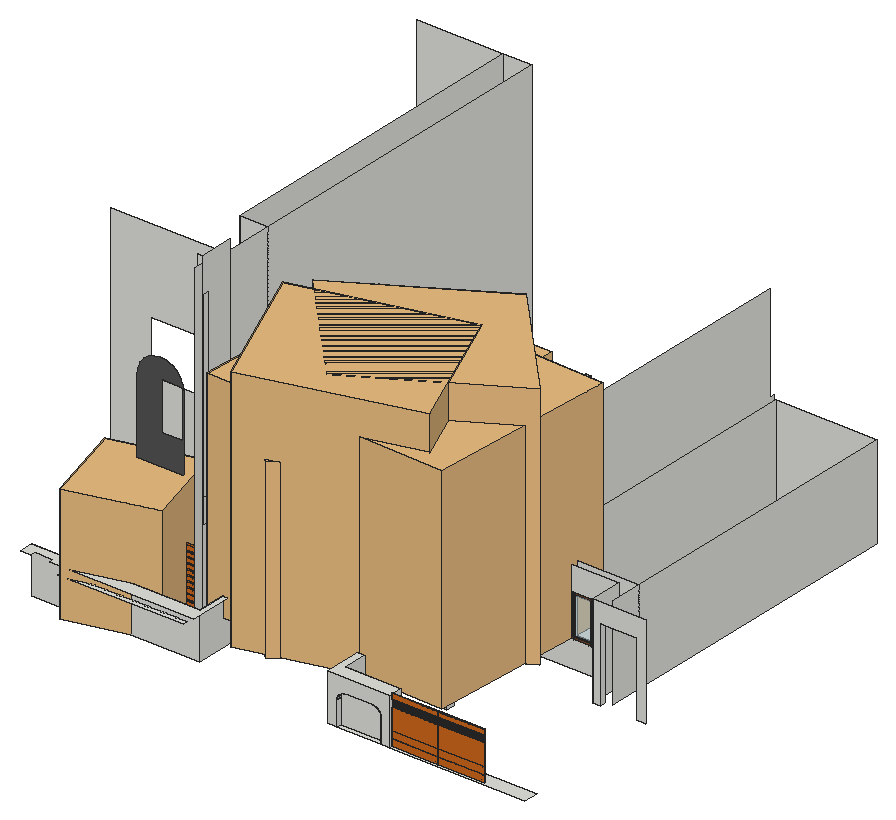
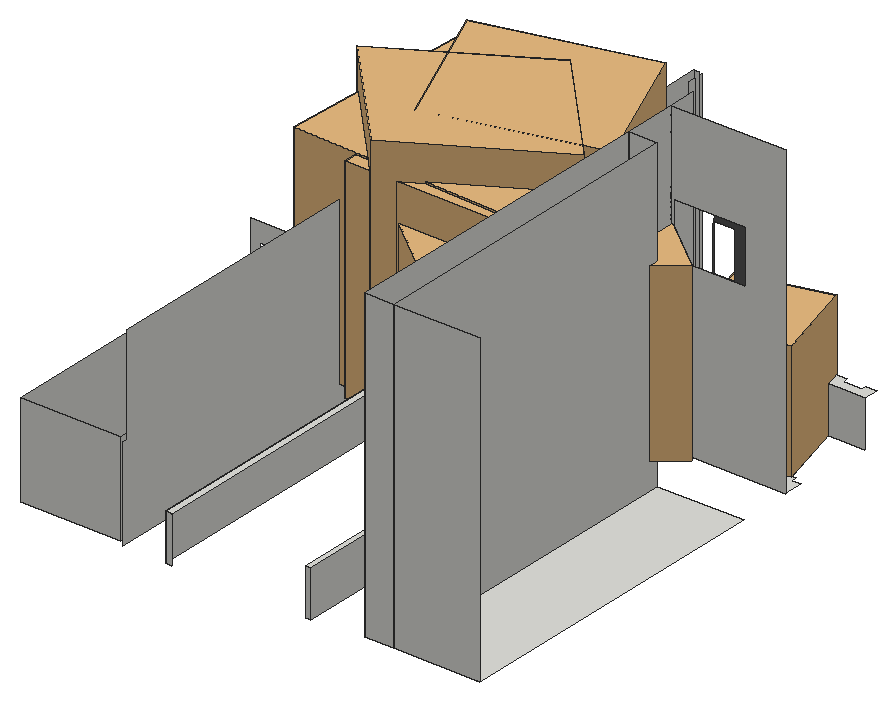
# SketchUp Ruby script. Lengths in inches.
U = 1.inch
M = Sketchup.active_model
def pt(a) = Geom::Point3d.new(a.map { |v| v * U })
def face(e, loops, mat)
  f = e.add_face(loops[0].map { |a| pt(a) })
  loops[1..].each { |l| e.add_face(l.map { |a| pt(a) }).erase! }
  f.material = f.back_material = mat if mat
  f
end
# faces: each face lists its corners as indices into pts; further lists are holes
def faces(e, pts, list, mat = nil) = list.each { |f| face(e, (f[0].is_a?(Array) ? f : [f]).map { |l| l.map { |i| pts[i] } }, mat) }
# xy, xz, yz: faces in a plane at the given z, y or x. An outline is a flat list of corners, or four numbers for a rectangle; further outlines are holes
def ring(l) = l.size == 4 ? [[l[0], l[1]], [l[2], l[1]], [l[2], l[3]], [l[0], l[3]]] : l.each_slice(2).to_a
def flat(e, list, mat, &to3) = list.each { |f| face(e, (f[0].is_a?(Array) ? f : [f]).map { |l| ring(l).map { |u, v| to3.(u, v) } }, mat) }
def xy(e, z, list, mat = nil) = flat(e, list, mat) { |x, y| [x, y, z] }
def xz(e, y, list, mat = nil) = flat(e, list, mat) { |x, z| [x, y, z] }
def yz(e, x, list, mat = nil) = flat(e, list, mat) { |y, z| [x, y, z] }
def lines(e, pts, list) = list.each { |a, b| e.add_line(pt(pts[a]), pt(pts[b])) }
# prism: a flat outline (further loops are holes) pulled along v
def prism(e, loops, v, mat = nil)
  f = face(e, loops, mat); d = Geom::Vector3d.new(v.map { |x| x * U })
  f.pushpull(f.normal.samedirection?(d) ? d.length : -d.length)
end
def box(e, o, s, mat = nil) = prism(e, [[o, [o[0] + s[0], o[1], o[2]], [o[0] + s[0], o[1] + s[1], o[2]], [o[0], o[1] + s[1], o[2]]]], [0, 0, s[2]], mat)
def at(x, y, z, deg = 0) = Geom::Transformation.translation(pt([x, y, z])) * Geom::Transformation.rotation(ORIGIN, Z_AXIS, deg.degrees)
def axes(o, x, y, z) = Geom::Transformation.new([*x, 0, *y, 0, *z, 0, *pt(o).to_a, 1])
def part(name) = M.definitions.add(name)
# library, detail: a bought-in or finely detailed component or shape, given as its bounding box
def library(name, o, s) = part(name).tap { |d| box(d.entities, o, s) }
def detail(e, o, s) = box(e.add_group.entities, o, s)
def put(e, d, t, mat = nil) = e.add_instance(d, t).tap { |i| i.material = mat if mat }
def group(e, t, mat = nil) = e.add_group.tap { |g| g.transformation = t; g.material = mat if mat }.entities
root = M.entities
M.materials.add("[0041_Chocolate]").color = [210, 105, 30]
M.materials.add("[Color M06]").color = [84, 84, 84]
M.materials.add("[Translucent Glass Safety]").color = [204, 235, 244]
M.materials["[Translucent Glass Safety]"].alpha = 0.5
M.materials.add("[Wood Veneer 01]").color = [120, 70, 37]
M.materials.add("[Wood Veneer 01]2").color = [94, 55, 29]
c1 = library("Palm tree",[-4.09,-4.52,0],[193.52,193.51,258.93])
c2 = part("Palm+Tree")
put(c2.entities,c1,at(25.51,-21.81,0,15))
c3 = library("Group\#287",[-33.32,-34.9375,32.67],[162.87,159.66,128.34])
c4 = library("Group\#288",[-10.45,-6.67,0],[121.7,116.61,164.95])
c5 = library("Group\#286",[-10.45,-6.67,0],[121.7,116.61,164.95])
c6 = library("Group\#284",[-10.45,-6.67,0],[121.7,116.61,164.95])
c7 = library("Group\#283",[-33.32,-34.9375,32.67],[162.87,159.66,128.34])
c8 = library("Group\#285",[-33.32,-34.9375,81.35],[162.87,159.66,79.66])
c9 = library("Group\#282",[-33.32,-34.9375,77.91],[162.87,159.66,83.1])
c10 = part("Palem Elek")
put(c10.entities,c3,axes([92.2,20.3,-29.73],[0.70711,0.70711,0],[-0.70711,0.70711,0],[0,0,0.91208]))
put(c10.entities,c4,axes([60.27,20.78,0],[1,0,0],[0,1,0],[0,0,0.85762]))
put(c10.entities,c5,at(25.45,60.83,0,-53.5))
put(c10.entities,c6,at(84.4375,135.48,0,-161.4))
put(c10.entities,c7,axes([38.54,105.7,-36.19],[-0.04013,-0.99919,0],[0.99919,-0.04013,0],[0,0,1.11001]))
put(c10.entities,c8,axes([57.15,96.51,-54.45],[-0.02003,-0.49872,0.02965],[0.4996,-0.02007,0],[0.00123,0.03065,0.51628]))
put(c10.entities,c9,axes([74.94,50.39,-54.06],[0.40095,0.29715,0.03075],[-0.29654,0.38966,0.10114],[0.04012,-0.11026,0.54246]))
c11 = part("palem elek\#1")
put(c11.entities,c10,at(-81.14,-74.56,-0.83))
c12 = part("Coqueiro")
put(c12.entities,c11,axes([83.17,89.39,9.5625],[0,1.1016,0],[-1.377,0,0],[0,0,1.39284]))
c13 = part("Slatted screen panel")
xy(c13.entities,0,[[0,0,255.91,1.97]],"[Wood Veneer 01]2")
xy(c13.entities,16.54,[[0,1.18,255.91,1.97]],"[Wood Veneer 01]2")
xy(c13.entities,16.93,[[0,0,255.91,1.18]],"[Wood Veneer 01]2")
xy(c13.entities,17.78,[[0,0,255.91,1.18]],"[Wood Veneer 01]2")
xy(c13.entities,34.45,[[0,0,255.91,1.18]],"[Wood Veneer 01]2")
xy(c13.entities,35.07,[[0,0,255.91,1.18]],"[Wood Veneer 01]2")
xy(c13.entities,89.37,[[0,0,255.91,1.97]],"[Wood Veneer 01]2")
xy(c13.entities,92.91,[[0,0,255.91,1.97]],"[Wood Veneer 01]2")
xy(c13.entities,94.49,[[0,0,255.91,1.97]],"[Wood Veneer 01]2")
xy(c13.entities,97.64,[[0,0,255.91,1.97]],"[Wood Veneer 01]2")
xy(c13.entities,99.21,[[0,0,255.91,1.97]],"[Wood Veneer 01]2")
xy(c13.entities,102.36,[[0,0,255.91,1.97]],"[Wood Veneer 01]2")
xy(c13.entities,103.9375,[[0,0,255.91,1.97]],"[Wood Veneer 01]2")
xy(c13.entities,107.48,[[0,0,255.91,1.97]],"[Wood Veneer 01]2")
xy(c13.entities,119.29,[[0,0,255.91,1.97]],"[Wood Veneer 01]2")
xz(c13.entities,0,[[0,0,255.91,16.93],[0,17.78,255.91,34.45],[0,35.07,255.91,89.37],[0,92.91,255.91,94.49],[0,97.64,255.91,99.21],
  [0,102.36,255.91,103.9375],[0,107.48,255.91,119.29]],"[0041_Chocolate]")
xz(c13.entities,1.18,[[0,16.54,255.91,16.93],[0,16.93,255.91,17.78],[0,34.45,255.91,35.07]],"[Wood Veneer 01]2")
xz(c13.entities,1.97,[[0,0,255.91,1.57],[0,1.57,255.91,5.51],[0,5.51,255.91,7.09],[0,7.09,255.91,11.8125],[0,11.8125,255.91,16.54],
  [0,16.54,255.91,19.69],[0,19.69,255.91,89.37],[0,92.91,255.91,94.49],[0,97.64,255.91,99.21],[0,102.36,255.91,103.9375],
  [0,107.48,255.91,109.84],[0,109.84,255.91,119.29]],"[Wood Veneer 01]2")
yz(c13.entities,0,[[0,0,1.97,1.57],[0,1.57,1.97,5.51],[0,5.51,1.97,7.09],[0,7.09,1.97,11.8125],[0,11.8125,0,16.93,1.18,16.93,1.18,16.54,1.97,16.54,1.97,11.8125],
  [1.18,16.54,1.97,19.69],[0,17.78,0,34.45,1.18,34.45,1.18,35.07,0,35.07,0,89.37,1.97,89.37,1.97,19.69,1.18,19.69,1.18,17.78],[0,92.91,1.97,94.49],[0,97.64,1.97,99.21],[0,102.36,1.97,103.9375],
  [0,107.48,1.97,109.84],[0,109.84,1.97,119.29]],"[Wood Veneer 01]2")
yz(c13.entities,255.91,[[0,0,1.97,1.57],[0,1.57,1.97,5.51],[0,5.51,1.97,7.09],[0,7.09,1.97,11.8125],[0,11.8125,1.97,11.8125,1.97,16.54,1.18,16.54,1.18,16.93,0,16.93],
  [1.18,16.54,1.97,19.69],[0,17.78,1.18,17.78,1.18,19.69,1.97,19.69,1.97,89.37,0,89.37,0,35.07,1.18,35.07,1.18,34.45,0,34.45],[0,92.91,1.97,94.49],[0,97.64,1.97,99.21],[0,102.36,1.97,103.9375],
  [0,107.48,1.97,109.84],[0,109.84,1.97,119.29]],"[Wood Veneer 01]2")
p = [[255.91,1.97,103.9375],[255.91,1.97,107.48],[0,1.97,107.48],[0,1.97,103.9375],[0,1.97,92.91],[0,1.97,89.37],
  [255.91,1.97,99.21],[255.91,1.97,102.36],[255.91,1.97,89.37],[255.91,1.97,92.91],[0,1.97,97.64],[0,1.97,94.49],
  [0,1.97,102.36],[0,1.97,99.21],[255.91,1.97,94.49],[255.91,1.97,97.64],[240.94,0,5.51],[240.94,1.97,5.51]]
lines(c13.entities,p,[[0,1],[2,3],[4,5],[6,7],[8,9],[10,11],[12,13],[14,15],[16,17]])
c14 = part("Group\#3")
g1 = group(c14.entities,at(0,0,0))
xy(g1,0,[[0,0,6,48]],"[Wood Veneer 01]")
xy(g1,4,[[0,4,1.8125,44],[1.8125,4,6,44]])
xy(g1,80,[[0,4,1.8125,44],[1.8125,4,6,44]])
xy(g1,84,[[0,0,6,48]],"[Wood Veneer 01]")
xz(g1,0,[[0,0,6,84]],"[Wood Veneer 01]")
xz(g1,4,[[0,4,1.8125,80],[1.8125,4,6,80]])
xz(g1,44,[[0,4,1.8125,80],[1.8125,4,6,80]])
xz(g1,48,[[0,0,6,84]],"[Wood Veneer 01]")
yz(g1,0,[[[0,0,48,84],[4,4,44,80]]],"[Wood Veneer 01]")
yz(g1,1.8125,[[4,4,44,80]],"[Translucent Glass Safety]")
yz(g1,6,[[[0,0,48,84],[4,4,44,80]]],"[Wood Veneer 01]")
g2 = group(c14.entities,at(0,48,0))
xy(g2,0,[[0,0,6,48]],"[Wood Veneer 01]")
xy(g2,4,[[0,4,1.8125,44],[1.8125,4,6,44]])
xy(g2,80,[[0,4,1.8125,44],[1.8125,4,6,44]])
xy(g2,84,[[0,0,6,48]],"[Wood Veneer 01]")
xz(g2,0,[[0,0,6,84]],"[Wood Veneer 01]")
xz(g2,4,[[0,4,1.8125,80],[1.8125,4,6,80]])
xz(g2,44,[[0,4,1.8125,80],[1.8125,4,6,80]])
xz(g2,48,[[0,0,6,84]],"[Wood Veneer 01]")
yz(g2,0,[[[0,0,48,84],[4,4,44,80]]],"[Wood Veneer 01]")
yz(g2,1.8125,[[4,4,44,80]],"[Translucent Glass Safety]")
yz(g2,6,[[[0,0,48,84],[4,4,44,80]]],"[Wood Veneer 01]")
xy(root,6.125,[[1898.05,198.625,1954.92,204.875],[1965.86,198.625,2140.66,217.125],[1547.71,280.47,1643.23,280.47,1643.23,292.45,1642.35,292.45,1642.35,302.0625,1547.71,302.0625],[1643.23,280.47,1649.14,292.45],[1547.21,292.45,1547.71,302.46],
  [1642.35,292.45,1643.23,302.46],[1643.23,292.45,1650.02,302.46],[1949.9,294.33,1962.9,305.58],[1547.71,302.0625,1642.35,302.46],[1547.71,302.46,1547.71,305.58,1507.74,305.58,1507.74,312.8125,1496.21,312.8125,1496.21,336.27,1643.23,336.27,1643.23,302.46],
  [1547.71,302.46,1547.71,305.58,1507.74,305.58,1507.74,312.8125,1547.71,312.8125,1547.71,305.58,1643.23,305.58,1643.23,302.46],[1547.21,302.46,1547.71,305.58],[1643.23,302.46,1650.02,305.58],[1643.23,305.58,1650.02,336.27],[1496.21,336.27,1643.23,337.5625],
  [1495.03,406.38,1606.23,830.91],[1606.23,406.38,1643.23,830.91],[1957.13,448.51,2087.21,830.91]])
xy(root,11.08,[[1547.71,280.47,1649.14,281.47]],"[0041_Chocolate]")
xy(root,13.1875,[[1547.71,280.47,1649.14,281.47]],"[0041_Chocolate]")
xy(root,18.14,[[1547.71,280.47,1649.14,281.47]],"[0041_Chocolate]")
xy(root,20.25,[[1547.71,280.47,1649.14,281.47]],"[0041_Chocolate]")
xy(root,25.2,[[1547.71,280.47,1649.14,281.47]],"[0041_Chocolate]")
xy(root,27.3125,[[1547.71,280.47,1649.14,281.47]],"[0041_Chocolate]")
xy(root,32.27,[[1547.71,280.47,1649.14,281.47]],"[0041_Chocolate]")
xy(root,34.375,[[1547.71,280.47,1649.14,281.47]],"[0041_Chocolate]")
xy(root,39.33,[[1547.71,280.47,1649.14,281.47]],"[0041_Chocolate]")
xy(root,40.13,[[1985.87,439.98,2033.5,448.51]])
xy(root,41.4375,[[1547.71,280.47,1649.14,281.47]],"[0041_Chocolate]")
xy(root,46.39,[[1547.71,280.47,1649.14,281.47]],"[0041_Chocolate]")
xy(root,48,[[1908.98,198.625,1943.43,204.875]])
xy(root,48.5,[[1547.71,280.47,1649.14,281.47]],"[0041_Chocolate]")
xy(root,53.45,[[1547.71,280.47,1649.14,281.47]],"[0041_Chocolate]")
xy(root,55.1875,[[1539,198.625,1539,203.875,1540.625,203.875,1540.625,204.875,1541.375,204.875,1541.375,203.875,1544.625,203.875,1544.625,204.875,1545.375,204.875,1545.375,203.875,1548.625,203.875,1548.625,204.875,1549.375,204.875,1549.375,203.875,1552.625,203.875,1552.625,204.875,1553.375,204.875,1553.375,203.875,1556.625,203.875,1556.625,204.875,1557.375,204.875,1557.375,203.875,1560.625,203.875,1560.625,204.875,1561.375,204.875,1561.375,203.875,1564.625,203.875,1564.625,204.875,1565.375,204.875,1565.375,203.875,1568.625,203.875,1568.625,204.875,1569.375,204.875,1569.375,203.875,1572.625,203.875,1572.625,204.875,1573.375,204.875,1573.375,203.875,1576.625,203.875,1576.625,204.875,1577.375,204.875,1577.375,203.875,1580.625,203.875,1580.625,204.875,1581.375,204.875,1581.375,203.875,1584.625,203.875,1584.625,204.875,1585.375,204.875,1585.375,203.875,1588.625,203.875,1588.625,204.875,1589.375,204.875,1589.375,203.875,1592.625,203.875,1592.625,204.875,1593.375,204.875,1593.375,203.875,1596.625,203.875,1596.625,204.875,1597.375,204.875,1597.375,203.875,1600.625,203.875,1600.625,204.875,1601.375,204.875,1601.375,203.875,1604.625,203.875,1604.625,204.875,1605.375,204.875,1605.375,203.875,1608.625,203.875,1608.625,204.875,1609.375,204.875,1609.375,203.875,1612.625,203.875,1612.625,204.875,1613.375,204.875,1613.375,203.875,1616.625,203.875,1616.625,204.875,1617.375,204.875,1617.375,203.875,1620.625,203.875,1620.625,204.875,1621.375,204.875,1621.375,203.875,1624.625,203.875,1624.625,204.875,1625.375,204.875,1625.375,203.875,1628.625,203.875,1628.625,204.875,1629.375,204.875,1629.375,203.875,1632.625,203.875,1632.625,204.875,1633.375,204.875,1633.375,203.875,1636.625,203.875,1636.625,204.875,1637.375,204.875,1637.375,203.875,1640.625,203.875,1640.625,204.875,1641.375,204.875,1641.375,203.875,1644.625,203.875,1644.625,204.875,1645.375,204.875,1645.375,203.875,1648.625,203.875,1648.625,204.875,1649.375,204.875,1649.375,203.875,1652.625,203.875,1652.625,204.875,1653.375,204.875,1653.375,203.875,1656.625,203.875,1656.625,204.875,1657.375,204.875,1657.375,203.875,1660.625,203.875,1660.625,204.875,1661.375,204.875,1661.375,203.875,1664.625,203.875,1664.625,204.875,1665.375,204.875,1665.375,203.875,1668.625,203.875,1668.625,204.875,1669.375,204.875,1669.375,203.875,1672.625,203.875,1672.625,204.875,1673.375,204.875,1673.375,203.875,1676.625,203.875,1676.625,204.875,1677.375,204.875,1677.375,203.875,1680.625,203.875,1680.625,204.875,1681.375,204.875,1681.375,203.875,1684.625,203.875,1684.625,204.875,1685.375,204.875,1685.375,203.875,1688.625,203.875,1688.625,204.875,1689.375,204.875,1689.375,203.875,1692.625,203.875,1692.625,204.875,1693.375,204.875,1693.375,203.875,1696.625,203.875,1696.625,204.875,1697.375,204.875,1697.375,203.875,1700.625,203.875,1700.625,198.625]])
xy(root,55.5625,[[1547.71,280.47,1649.14,281.47]],"[0041_Chocolate]")
xy(root,60.52,[[1547.71,280.47,1649.14,281.47]],"[0041_Chocolate]")
xy(root,62.625,[[1547.71,280.47,1649.14,281.47]],"[0041_Chocolate]")
xy(root,66.125,[[1490.16,198.625,1503.29,198.625,1503.29,204.875,1527.6,204.875,1527.6,198.625,1713.52,198.625,1713.52,838.14,1707,838.14,1707,217.125,1490.16,217.125],[1886.4,198.625,1965.86,198.625,1965.86,217.125,1894.57,217.125,1894.57,838.14,1886.4,838.14]])
xy(root,67.58,[[1547.71,280.47,1649.14,281.47]],"[0041_Chocolate]")
xy(root,69.6875,[[1547.71,280.47,1649.14,281.47]],"[0041_Chocolate]")
xy(root,74.64,[[1547.71,280.47,1583.91,281.47],[1601.86,280.47,1649.14,281.47]],"[0041_Chocolate]")
xy(root,76.75,[[1547.71,280.47,1578.82,281.47],[1606.95,280.47,1649.14,281.47]],"[0041_Chocolate]")
xy(root,81.7,[[1547.71,280.47,1571.98,281.47],[1613.79,280.47,1649.14,281.47]],"[0041_Chocolate]")
xy(root,83.8125,[[1547.71,280.47,1570.3,281.47],[1615.47,280.47,1649.14,281.47]],"[0041_Chocolate]")
xy(root,88.77,[[1547.71,280.47,1566.77,281.47],[1619,280.47,1649.14,281.47]],"[0041_Chocolate]")
xz(root,198.625,[[1886.4,6.125,1898.05,6.125,1898.05,37.07,1898.14,38.5,1898.42,39.9,1898.88,41.25,1899.51,42.53,1900.31,43.72,1901.25,44.8,1902.32,45.74,1903.51,46.54,1904.8,47.17,1906.15,47.63,1907.55,47.91,1908.98,48,1943.43,48,1944.93,47.9,1946.4,47.61,1947.83,47.125,1949.18,46.46,1950.43,45.625,1951.56,44.63,1952.55,43.5,1953.38,42.25,1954.05,40.9,1954.53,39.48,1954.82,38.01,1954.92,36.51,1954.92,6.125,1965.86,6.125,1965.86,66.125,1886.4,66.125]])
xz(root,204.875,[[1898.05,6.125,1954.92,6.125,1954.92,36.51,1954.82,38.01,1954.53,39.48,1954.05,40.9,1953.38,42.25,1952.55,43.5,1951.56,44.63,1950.43,45.625,1949.18,46.46,1947.83,47.125,1946.4,47.61,1944.93,47.9,1943.43,48,1908.98,48,1907.55,47.91,1906.15,47.63,1904.8,47.17,1903.51,46.54,1902.32,45.74,1901.25,44.8,1900.31,43.72,1899.51,42.53,1898.88,41.25,1898.42,39.9,1898.14,38.5,1898.05,37.07]])
xz(root,217.125,[[1490.16,6.125,1707,66.125],[1894.57,6.125,1965.86,66.125]])
xz(root,280.47,[[1547.71,6.125,1649.14,11.08],[1547.71,13.1875,1649.14,18.14],[1547.71,20.25,1649.14,25.2],[1547.71,27.3125,1649.14,32.27],[1547.71,34.375,1649.14,39.33],
  [1547.71,41.4375,1649.14,46.39],[1547.71,48.5,1649.14,53.45],[1547.71,55.5625,1649.14,60.52],[1547.71,62.625,1649.14,67.58],[1547.71,69.6875,1649.14,69.6875,1649.14,74.64,1601.86,74.64,1600.59,74.12,1592.88,73.1,1585.17,74.12,1583.91,74.64,1547.71,74.64],
  [1547.71,76.75,1578.82,76.75,1577.99,77.09,1571.98,81.7,1547.71,81.7],[1606.95,76.75,1649.14,76.75,1649.14,81.7,1613.79,81.7,1607.78,77.09],[1547.71,83.8125,1570.3,83.8125,1567.09,88,1566.77,88.77,1547.71,88.77],[1615.47,83.8125,1649.14,83.8125,1649.14,88.77,1619,88.77,1618.68,88]],"[0041_Chocolate]")
xz(root,281.47,[[1547.71,11.08,1649.14,13.1875],[1547.71,18.14,1649.14,20.25],[1547.71,25.2,1649.14,27.3125],[1547.71,32.27,1649.14,34.375],[1547.71,39.33,1649.14,41.4375],
  [1547.71,46.39,1649.14,48.5],[1547.71,53.45,1649.14,55.5625],[1547.71,60.52,1649.14,62.625],[1547.71,67.58,1649.14,69.6875],[1547.71,74.64,1583.91,74.64,1578.82,76.75,1547.71,76.75],
  [1601.86,74.64,1649.14,74.64,1649.14,76.75,1606.95,76.75],[1547.71,81.7,1571.98,81.7,1571.82,81.83,1570.3,83.8125,1547.71,83.8125],[1613.79,81.7,1649.14,81.7,1649.14,83.8125,1615.47,83.8125,1613.95,81.83],[1547.71,88.77,1566.77,88.77,1565.89,90.875,1547.71,90.875],[1619,88.77,1649.14,88.77,1649.14,90.875,1619.87,90.875]],"[0041_Chocolate]")
xz(root,292.45,[[1642.35,6.125,1643.23,126.125],[1643.23,6.125,1649.14,126.125],[1649.14,6.125,1650.02,6.125,1650.02,421.25,1643.23,421.25,1643.23,141.26,1649.14,141.26]])
xz(root,294.33,[[1949.9,6.125,1962.9,128.75]])
xz(root,295.65,[[[1592.88,73.1,1600.59,74.12,1601.86,74.64,1606.95,76.75,1607.78,77.09,1613.79,81.7,1613.95,81.83,1615.47,83.8125,1618.68,88,1619,88.77,1619.87,90.875,1621.66,95.18,1621.74,95.83,1621.93,97.27,1597.48,97.27,1597.48,145.27,1622.67,145.27,1622.67,253.3125,1622.02,258.27,1621.74,260.375,1621.66,261.02,1619.87,265.33,1619,267.4375,1618.68,268.21,1615.47,272.39,1613.95,274.375,1613.79,274.5,1607.78,279.11,1606.95,279.45,1601.86,281.5625,1600.59,282.09,1592.88,283.1,1585.17,282.09,1583.91,281.5625,1578.82,279.45,1577.99,279.11,1571.98,274.5,1571.82,274.375,1570.3,272.39,1567.09,268.21,1566.77,267.4375,1565.89,265.33,1564.11,261.02,1564.03,260.375,1563.75,258.27,1563.1,253.3125,1563.1,102.89,1563.75,97.9375,1564.03,95.83,1564.11,95.18,1565.89,90.875,1566.77,88.77,1567.09,88,1570.3,83.8125,1571.82,81.83,1571.98,81.7,1577.99,77.09,1578.82,76.75,1583.91,74.64,1585.17,74.12],[1595.33,196.89,1622.02,258.27]]],"[Color M06]")
xz(root,302.46,[[1547.71,6.125,1634.68,8.32],[1634.68,6.125,1642.35,8.32],[1642.35,6.125,1643.23,8.32],[1643.23,6.125,1650.02,8.32],[1547.71,8.32,1634.68,126.125],
  [1634.68,8.32,1642.35,109.9375],[1642.35,8.32,1643.23,109.9375]])
xz(root,305.58,[[1949.9,6.125,1962.9,128.75]])
xz(root,337.5625,[[[1496.21,6.125,1643.23,402.64],[1547.71,226.8,1640.52,295.72]]])
xz(root,397.86,[[2068.38,6.125,2078.42,6.125,2078.42,101.1875,2125.61,101.1875,2125.61,6.125,2137,6.125,2137,126.125,2068.38,126.125]])
xz(root,406.38,[[1606.23,6.125,1643.23,402.64]])
xz(root,439.98,[[[1949.9,6.125,2068.38,126.125],[1985.87,40.13,2033.5,95.51]]])
xz(root,448.51,[[1957.13,6.125,1965.65,126.125],[[1965.65,6.125,2087.21,126.125],[1985.87,40.13,2033.5,95.51]]])
xz(root,830.91,[[1495.03,6.125,1606.23,402.64],[1606.23,6.125,1643.23,402.64],[1957.13,6.125,2087.21,126.125]])
xz(root,838.14,[[1707,6.125,1713.52,66.125],[1886.4,6.125,1894.57,66.125]])
yz(root,1547.71,[[280.47,6.125,280.47,11.08,281.47,11.08,281.47,13.1875,280.47,13.1875,280.47,18.14,281.47,18.14,281.47,20.25,280.47,20.25,280.47,25.2,281.47,25.2,281.47,27.3125,280.47,27.3125,280.47,32.27,281.47,32.27,281.47,34.375,280.47,34.375,280.47,39.33,281.47,39.33,281.47,41.4375,280.47,41.4375,280.47,46.39,281.47,46.39,281.47,48.5,280.47,48.5,280.47,53.45,281.47,53.45,281.47,55.5625,280.47,55.5625,280.47,60.52,281.47,60.52,281.47,62.625,280.47,62.625,280.47,67.58,281.47,67.58,281.47,69.6875,280.47,69.6875,280.47,74.64,281.47,74.64,281.47,76.75,280.47,76.75,280.47,81.7,281.47,81.7,281.47,83.8125,280.47,83.8125,280.47,88.77,281.47,88.77,281.47,90.875,280.47,90.875,280.47,95.83,281.47,95.83,281.47,97.9375,280.47,97.9375,280.47,102.89,281.47,102.89,281.47,105,280.47,105,280.47,109.95,281.47,109.95,281.47,112.0625,280.47,112.0625,280.47,117.02,281.47,117.02,281.47,119.125,280.47,119.125,280.47,124.08,281.47,124.08,281.47,126.1875,280.47,126.1875,280.47,131.14,281.47,131.14,281.47,133.25,280.47,133.25,280.47,138.2,281.47,138.2,281.47,140.3125,280.47,140.3125,280.47,141.26,292.45,141.26,292.45,126.125,302.46,126.125,302.46,6.125]])
yz(root,1606.23,[[406.38,6.125,830.91,402.64]])
yz(root,1642.35,[[292.45,6.125,302.46,126.125]])
yz(root,1643.23,[[302.46,6.125,337.5625,402.64],[337.5625,6.125,406.38,402.64],[406.38,6.125,830.91,402.64]])
yz(root,1649.14,[[280.47,6.125,292.45,6.125,292.45,141.26,302.46,141.26,302.46,411.82,281.47,411.82,281.47,405.64,280.47,405.64,280.47,400.6875,281.47,400.6875,281.47,398.77,280.47,398.77,280.47,393.8125,281.47,393.8125,281.47,391.89,280.47,391.89,280.47,386.9375,281.47,386.9375,281.47,385.02,280.47,385.02,280.47,380.0625,281.47,380.0625,281.47,378.14,280.47,378.14,280.47,373.1875,281.47,373.1875,281.47,371.27,280.47,371.27,280.47,366.3125,281.47,366.3125,281.47,364.2,280.47,364.2,280.47,359.25,281.47,359.25,281.47,357.14,280.47,357.14,280.47,352.1875,281.47,352.1875,281.47,350.08,280.47,350.08,280.47,345.125,281.47,345.125,281.47,343.02,280.47,343.02,280.47,338.0625,281.47,338.0625,281.47,335.95,280.47,335.95,280.47,331,281.47,331,281.47,328.89,280.47,328.89,280.47,323.9375,281.47,323.9375,281.47,321.83,280.47,321.83,280.47,316.875,281.47,316.875,281.47,314.77,280.47,314.77,280.47,309.8125,281.47,309.8125,281.47,307.7,280.47,307.7,280.47,302.75,281.47,302.75,281.47,300.64,280.47,300.64,280.47,295.6875,281.47,295.6875,281.47,293.58,280.47,293.58,280.47,288.625,281.47,288.625,281.47,286.52,280.47,286.52,280.47,281.5625,281.47,281.5625,281.47,279.45,280.47,279.45,280.47,274.5,281.47,274.5,281.47,272.39,280.47,272.39,280.47,267.4375,281.47,267.4375,281.47,265.33,280.47,265.33,280.47,260.375,281.47,260.375,281.47,258.27,280.47,258.27,280.47,253.3125,281.47,253.3125,281.47,251.2,280.47,251.2,280.47,246.25,281.47,246.25,281.47,244.14,280.47,244.14,280.47,239.1875,281.47,239.1875,281.47,237.08,280.47,237.08,280.47,232.125,281.47,232.125,281.47,230.02,280.47,230.02,280.47,225.0625,281.47,225.0625,281.47,222.95,280.47,222.95,280.47,218,281.47,218,281.47,215.89,280.47,215.89,280.47,210.9375,281.47,210.9375,281.47,208.83,280.47,208.83,280.47,203.875,281.47,203.875,281.47,201.77,280.47,201.77,280.47,196.8125,281.47,196.8125,281.47,194.7,280.47,194.7,280.47,189.75,281.47,189.75,281.47,187.64,280.47,187.64,280.47,182.6875,281.47,182.6875,281.47,180.58,280.47,180.58,280.47,175.625,281.47,175.625,281.47,173.52,280.47,173.52,280.47,168.5625,281.47,168.5625,281.47,166.45,280.47,166.45,280.47,161.5,281.47,161.5,281.47,159.39,280.47,159.39,280.47,154.4375,281.47,154.4375,281.47,152.33,280.47,152.33,280.47,147.375,281.47,147.375,281.47,145.27,280.47,145.27,280.47,140.3125,281.47,140.3125,281.47,138.2,280.47,138.2,280.47,133.25,281.47,133.25,281.47,131.14,280.47,131.14,280.47,126.1875,281.47,126.1875,281.47,124.08,280.47,124.08,280.47,119.125,281.47,119.125,281.47,117.02,280.47,117.02,280.47,112.0625,281.47,112.0625,281.47,109.95,280.47,109.95,280.47,105,281.47,105,281.47,102.89,280.47,102.89,280.47,97.9375,281.47,97.9375,281.47,95.83,280.47,95.83,280.47,90.875,281.47,90.875,281.47,88.77,280.47,88.77,280.47,83.8125,281.47,83.8125,281.47,81.7,280.47,81.7,280.47,76.75,281.47,76.75,281.47,74.64,280.47,74.64,280.47,69.6875,281.47,69.6875,281.47,67.58,280.47,67.58,280.47,62.625,281.47,62.625,281.47,60.52,280.47,60.52,280.47,55.5625,281.47,55.5625,281.47,53.45,280.47,53.45,280.47,48.5,281.47,48.5,281.47,46.39,280.47,46.39,280.47,41.4375,281.47,41.4375,281.47,39.33,280.47,39.33,280.47,34.375,281.47,34.375,281.47,32.27,280.47,32.27,280.47,27.3125,281.47,27.3125,281.47,25.2,280.47,25.2,280.47,20.25,281.47,20.25,281.47,18.14,280.47,18.14,280.47,13.1875,281.47,13.1875,281.47,11.08,280.47,11.08]])
yz(root,1650.02,[[292.45,6.125,336.27,6.125,336.27,421.25,292.45,421.25,292.45,376.875,302.46,376.875,302.46,109.9375,299.11,109.9375,295.02,110.21,292.45,110.72]])
yz(root,1707,[[217.125,6.125,838.14,66.125]])
yz(root,1894.57,[[217.125,6.125,838.14,66.125]])
yz(root,1898.05,[[198.625,6.125,204.875,37.07]])
yz(root,1949.9,[[294.33,6.125,294.33,128.75,298.39,128.75,298.39,126.125,305.58,126.125,305.58,6.125],[439.98,6.125,439.98,252.47,830.91,252.47,830.91,126.125,838.14,126.125,838.14,6.125]])
yz(root,1954.92,[[198.625,6.125,204.875,36.51]])
yz(root,1957.13,[[448.51,6.125,830.91,126.125]])
yz(root,1962.9,[[294.33,6.125,305.58,128.75]])
yz(root,1965.86,[[198.625,6.125,217.125,66.125]])
yz(root,1985.87,[[439.98,40.13,448.51,95.51]])
yz(root,2033.5,[[439.98,40.13,448.51,95.51]])
yz(root,2068.38,[[397.86,6.125,439.98,126.125]])
yz(root,2078.42,[[397.86,6.125,405.05,101.1875]])
yz(root,2087.21,[[406.38,6.125,448.51,126.125],[448.51,6.125,830.91,126.125]])
p = [[1954.82,204.875,38.01],[1954.92,204.875,36.51],[1954.92,198.625,36.51],[1954.82,198.625,38.01],[1898.05,204.875,37.07],[1898.14,204.875,38.5],
  [1898.14,198.625,38.5],[1898.05,198.625,37.07],[1954.53,204.875,39.48],[1954.53,198.625,39.48],[1898.42,204.875,39.9],[1898.42,198.625,39.9],
  [1954.05,204.875,40.9],[1954.05,198.625,40.9],[1898.88,204.875,41.25],[1898.88,198.625,41.25],[1953.38,204.875,42.25],[1953.38,198.625,42.25],
  [1899.51,204.875,42.53],[1899.51,198.625,42.53],[1952.55,204.875,43.5],[1952.55,198.625,43.5],[1900.31,204.875,43.72],[1900.31,198.625,43.72],
  [1951.56,204.875,44.63],[1951.56,198.625,44.63],[1901.25,204.875,44.8],[1901.25,198.625,44.8],[1950.43,204.875,45.625],[1950.43,198.625,45.625],
  [1902.32,204.875,45.74],[1902.32,198.625,45.74],[1949.18,204.875,46.46],[1949.18,198.625,46.46],[1903.51,204.875,46.54],[1903.51,198.625,46.54],
  [1904.8,204.875,47.17],[1904.8,198.625,47.17],[1947.83,204.875,47.125],[1947.83,198.625,47.125],[1946.4,204.875,47.61],[1946.4,198.625,47.61],
  [1906.15,204.875,47.63],[1906.15,198.625,47.63],[1907.55,204.875,47.91],[1907.55,198.625,47.91],[1944.93,204.875,47.9],[1944.93,198.625,47.9],
  [1908.98,204.875,48],[1908.98,198.625,48],[1943.43,204.875,48],[1943.43,198.625,48],[1585.17,295.65,74.12],[1585.17,280.47,74.12],
  [1592.88,280.47,73.1],[1592.88,295.65,73.1],[1600.59,280.47,74.12],[1600.59,295.65,74.12],[1583.91,295.65,74.64],[1583.91,281.47,74.64],
  [1583.91,280.47,74.64],[1601.86,280.47,74.64],[1601.86,281.47,74.64],[1601.86,295.65,74.64],[1578.82,281.47,76.75],[1578.82,295.65,76.75],
  [1606.95,281.47,76.75],[1606.95,295.65,76.75],[1577.99,295.65,77.09],[1577.99,280.47,77.09],[1578.82,280.47,76.75],[1606.95,280.47,76.75],
  [1607.78,280.47,77.09],[1607.78,295.65,77.09],[1571.98,295.65,81.7],[1571.98,281.47,81.7],[1571.98,280.47,81.7],[1613.79,280.47,81.7],
  [1613.79,281.47,81.7],[1613.79,295.65,81.7],[1571.82,281.47,81.83],[1571.82,295.65,81.83],[1613.95,281.47,81.83],[1613.95,295.65,81.83],
  [1570.3,281.47,83.8125],[1570.3,295.65,83.8125],[1615.47,281.47,83.8125],[1615.47,295.65,83.8125],[1567.09,295.65,88],[1567.09,280.47,88],
  [1570.3,280.47,83.8125],[1615.47,280.47,83.8125],[1618.68,280.47,88],[1618.68,295.65,88],[1566.77,295.65,88.77],[1566.77,281.47,88.77],
  [1566.77,280.47,88.77],[1619,280.47,88.77],[1619,281.47,88.77],[1619,295.65,88.77],[1565.89,281.47,90.875],[1565.89,295.65,90.875],
  [1619.87,281.47,90.875],[1619.87,295.65,90.875],[1547.71,312.8125,24.125],[1547.71,312.8125,6.125],[1547.71,321.34,24.125]]
faces(root,p,[[0,1,2,3],[4,5,6,7],[8,0,3,9],[5,10,11,6],[12,8,9,13],[10,14,15,11],[16,12,13,17],[14,18,19,15],
  [20,16,17,21],[18,22,23,19],[24,20,21,25],[22,26,27,23],[28,24,25,29],[26,30,31,27],[32,28,29,33],[30,34,35,31],
  [34,36,37,35],[38,32,33,39],[40,38,39,41],[36,42,43,37],[42,44,45,43],[46,40,41,47],[44,48,49,45],[50,46,47,51]])
faces(root,p,[[52,53,54,55],[55,54,56,57],[58,59,60,53,52],[57,56,61,62,63],[64,59,58,65],[62,66,67,63],[68,69,70,64,65],[67,66,71,72,73],
  [74,75,76,69,68],[73,72,77,78,79],[80,75,74,81],[78,82,83,79],[84,80,81,85],[82,86,87,83],[88,89,90,84,85],[87,86,91,92,93],
  [94,95,96,89,88],[93,92,97,98,99],[100,95,94,101],[98,102,103,99]],"[Color M06]")
lines(root,p,[[104,105],[104,106]])
put(root,c2,axes([1529.61,212.94,6.125],[0.58344,0,0],[0,0.58344,0],[0,0,0.58344]),"[Color M06]")
put(root,c12,axes([1696.82,246.74,29.13],[1.38444,0,0],[0,1.38444,0],[0,0,1.38444]))
put(root,c13,axes([1965.96,201.88,6.125],[0.23355,0,0],[0,0.5124,0],[0,0,0.5124]),"[0041_Chocolate]")
put(root,c14,axes([1985.87,442.86,40.13],[0,-0.48,0],[0.49609,0,0],[0,0,0.65923]))
put(root,c13,axes([2025.73,201.88,6.125],[0.23355,0,0],[0,0.5124,0],[0,0,0.5124]),"[0041_Chocolate]")
